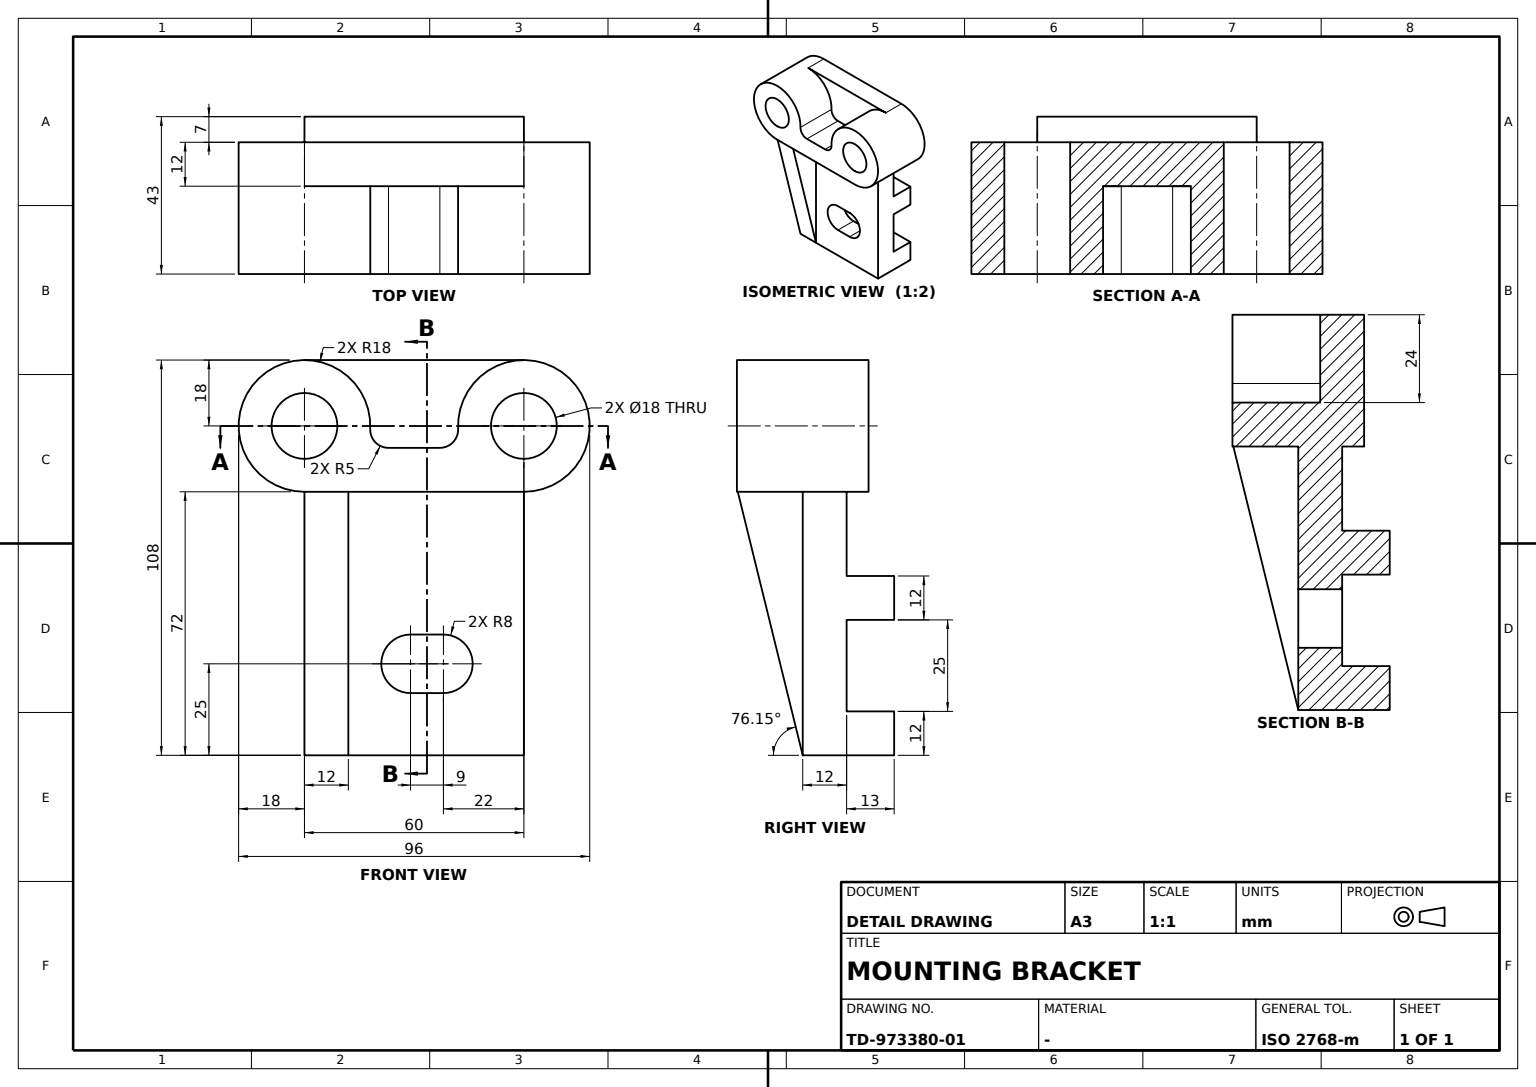
ISO-10303-21;
HEADER;
FILE_DESCRIPTION((''),'2;1');
FILE_NAME('','',(''),(''),'','','');
FILE_SCHEMA(('AUTOMOTIVE_DESIGN'));
ENDSEC;
DATA;
#1=APPLICATION_CONTEXT('');
#2=PRODUCT_CONTEXT('',#1,'mechanical');
#3=PRODUCT('','','',(#2));
#4=PRODUCT_DEFINITION_FORMATION('','',#3);
#5=PRODUCT_DEFINITION_CONTEXT('',#1,'design');
#6=PRODUCT_DEFINITION('','',#4,#5);
#7=PRODUCT_DEFINITION_SHAPE('','',#6);
#8=(LENGTH_UNIT()NAMED_UNIT(*)SI_UNIT(.MILLI.,.METRE.));
#9=(NAMED_UNIT(*)PLANE_ANGLE_UNIT()SI_UNIT($,.RADIAN.));
#10=(NAMED_UNIT(*)SI_UNIT($,.STERADIAN.)SOLID_ANGLE_UNIT());
#11=UNCERTAINTY_MEASURE_WITH_UNIT(LENGTH_MEASURE(0.005),#8,'distance_accuracy_value','');
#12=(GEOMETRIC_REPRESENTATION_CONTEXT(3)GLOBAL_UNCERTAINTY_ASSIGNED_CONTEXT((#11))GLOBAL_UNIT_ASSIGNED_CONTEXT((#8,#9,#10))REPRESENTATION_CONTEXT('',''));
#13=CARTESIAN_POINT('',(-18.,30.,45.));
#14=VERTEX_POINT('',#13);
#15=CARTESIAN_POINT('',(-18.,30.,54.));
#16=DIRECTION('',(1.,0.,0.));
#17=DIRECTION('',(0.,0.,-1.));
#18=AXIS2_PLACEMENT_3D('',#15,#16,#17);
#19=CIRCLE('',#18,9.);
#20=EDGE_CURVE('',#14,#14,#19,.T.);
#21=ORIENTED_EDGE('',*,*,#20,.F.);
#22=EDGE_LOOP('',(#21));
#23=FACE_BOUND('',#22,.T.);
#24=CARTESIAN_POINT('',(18.,30.,45.));
#25=VERTEX_POINT('',#24);
#26=CARTESIAN_POINT('',(18.,30.,54.));
#27=AXIS2_PLACEMENT_3D('',#26,#16,#17);
#28=CIRCLE('',#27,9.);
#29=EDGE_CURVE('',#25,#25,#28,.T.);
#30=ORIENTED_EDGE('',*,*,#29,.T.);
#31=EDGE_LOOP('',(#30));
#32=FACE_BOUND('',#31,.T.);
#33=CARTESIAN_POINT('',(0.,30.,54.));
#34=DIRECTION('',(0.,1.,0.));
#35=AXIS2_PLACEMENT_3D('',#33,#16,#34);
#36=CYLINDRICAL_SURFACE('',#35,9.);
#37=ADVANCED_FACE('',(#23,#32),#36,.F.);
#38=CARTESIAN_POINT('',(0.,-1.,-19.));
#39=VERTEX_POINT('',#38);
#40=CARTESIAN_POINT('',(0.,8.,-19.));
#41=VERTEX_POINT('',#40);
#42=CARTESIAN_POINT('',(0.,0.,-19.));
#43=VECTOR('',#34,1000.);
#44=LINE('',#42,#43);
#45=EDGE_CURVE('',#39,#41,#44,.T.);
#46=ORIENTED_EDGE('',*,*,#45,.T.);
#47=CARTESIAN_POINT('',(-12.,8.,-19.));
#48=VERTEX_POINT('',#47);
#49=CARTESIAN_POINT('',(-13.16,8.,-19.));
#50=VECTOR('',#16,1000.);
#51=LINE('',#49,#50);
#52=EDGE_CURVE('',#41,#48,#51,.F.);
#53=ORIENTED_EDGE('',*,*,#52,.T.);
#54=CARTESIAN_POINT('',(-12.,-1.,-19.));
#55=VERTEX_POINT('',#54);
#56=LINE('',#54,#43);
#57=EDGE_CURVE('',#55,#48,#56,.T.);
#58=ORIENTED_EDGE('',*,*,#57,.F.);
#59=CARTESIAN_POINT('',(-13.16,-1.,-19.));
#60=LINE('',#59,#50);
#61=EDGE_CURVE('',#39,#55,#60,.F.);
#62=ORIENTED_EDGE('',*,*,#61,.F.);
#63=EDGE_LOOP('',(#46,#53,#58,#62));
#64=FACE_BOUND('',#63,.T.);
#65=DIRECTION('',(0.,0.,1.));
#66=AXIS2_PLACEMENT_3D('',#38,#65,#34);
#67=PLANE('',#66);
#68=ADVANCED_FACE('',(#64),#67,.T.);
#69=CARTESIAN_POINT('',(-12.,-30.,13.));
#70=VERTEX_POINT('',#69);
#71=CARTESIAN_POINT('',(-25.,-30.,13.));
#72=VERTEX_POINT('',#71);
#73=CARTESIAN_POINT('',(0.,-30.,13.));
#74=DIRECTION('',(-1.,0.,0.));
#75=VECTOR('',#74,1000.);
#76=LINE('',#73,#75);
#77=EDGE_CURVE('',#70,#72,#76,.T.);
#78=ORIENTED_EDGE('',*,*,#77,.T.);
#79=CARTESIAN_POINT('',(-25.,-30.,1.));
#80=VERTEX_POINT('',#79);
#81=CARTESIAN_POINT('',(-25.,-30.,0.));
#82=VECTOR('',#17,1000.);
#83=LINE('',#81,#82);
#84=EDGE_CURVE('',#72,#80,#83,.T.);
#85=ORIENTED_EDGE('',*,*,#84,.T.);
#86=CARTESIAN_POINT('',(-12.,-30.,1.));
#87=VERTEX_POINT('',#86);
#88=CARTESIAN_POINT('',(0.,-30.,1.));
#89=LINE('',#88,#50);
#90=EDGE_CURVE('',#80,#87,#89,.T.);
#91=ORIENTED_EDGE('',*,*,#90,.T.);
#92=CARTESIAN_POINT('',(-12.,-30.,-24.));
#93=VERTEX_POINT('',#92);
#94=CARTESIAN_POINT('',(-12.,-30.,0.));
#95=LINE('',#94,#82);
#96=EDGE_CURVE('',#87,#93,#95,.T.);
#97=ORIENTED_EDGE('',*,*,#96,.T.);
#98=CARTESIAN_POINT('',(-25.,-30.,-24.));
#99=VERTEX_POINT('',#98);
#100=CARTESIAN_POINT('',(0.,-30.,-24.));
#101=LINE('',#100,#75);
#102=EDGE_CURVE('',#93,#99,#101,.T.);
#103=ORIENTED_EDGE('',*,*,#102,.T.);
#104=CARTESIAN_POINT('',(-25.,-30.,-36.));
#105=VERTEX_POINT('',#104);
#106=EDGE_CURVE('',#99,#105,#83,.T.);
#107=ORIENTED_EDGE('',*,*,#106,.T.);
#108=CARTESIAN_POINT('',(0.,-30.,-36.));
#109=VERTEX_POINT('',#108);
#110=LINE('',#108,#50);
#111=EDGE_CURVE('',#105,#109,#110,.T.);
#112=ORIENTED_EDGE('',*,*,#111,.T.);
#113=CARTESIAN_POINT('',(17.753425,-30.,36.));
#114=VERTEX_POINT('',#113);
#115=CARTESIAN_POINT('',(8.367946,-30.,-2.063329));
#116=DIRECTION('',(-0.239404888,0.,-0.970919822));
#117=VECTOR('',#116,1000.);
#118=LINE('',#115,#117);
#119=EDGE_CURVE('',#114,#109,#118,.T.);
#120=ORIENTED_EDGE('',*,*,#119,.F.);
#121=CARTESIAN_POINT('',(-12.,-30.,36.));
#122=VERTEX_POINT('',#121);
#123=CARTESIAN_POINT('',(0.,-30.,36.));
#124=LINE('',#123,#50);
#125=EDGE_CURVE('',#122,#114,#124,.T.);
#126=ORIENTED_EDGE('',*,*,#125,.F.);
#127=EDGE_CURVE('',#122,#70,#95,.T.);
#128=ORIENTED_EDGE('',*,*,#127,.T.);
#129=EDGE_LOOP('',(#78,#85,#91,#97,#103,#107,#112,#120,#126,#128));
#130=FACE_BOUND('',#129,.T.);
#131=CARTESIAN_POINT('',(0.,-30.,0.));
#132=AXIS2_PLACEMENT_3D('',#131,#34,#74);
#133=PLANE('',#132);
#134=ADVANCED_FACE('',(#130),#133,.F.);
#135=CARTESIAN_POINT('',(-18.,30.,36.));
#136=VERTEX_POINT('',#135);
#137=CARTESIAN_POINT('',(-12.,30.,36.));
#138=VERTEX_POINT('',#137);
#139=CARTESIAN_POINT('',(0.,30.,36.));
#140=LINE('',#139,#50);
#141=EDGE_CURVE('',#136,#138,#140,.T.);
#142=ORIENTED_EDGE('',*,*,#141,.T.);
#143=CARTESIAN_POINT('',(-12.,0.,36.));
#144=LINE('',#143,#43);
#145=EDGE_CURVE('',#122,#138,#144,.T.);
#146=ORIENTED_EDGE('',*,*,#145,.F.);
#147=CARTESIAN_POINT('',(-18.,-30.,36.));
#148=VERTEX_POINT('',#147);
#149=EDGE_CURVE('',#148,#122,#124,.T.);
#150=ORIENTED_EDGE('',*,*,#149,.F.);
#151=CARTESIAN_POINT('',(-18.,0.,36.));
#152=LINE('',#151,#43);
#153=EDGE_CURVE('',#148,#136,#152,.T.);
#154=ORIENTED_EDGE('',*,*,#153,.T.);
#155=EDGE_LOOP('',(#142,#146,#150,#154));
#156=FACE_BOUND('',#155,.T.);
#157=CARTESIAN_POINT('',(0.,0.,36.));
#158=AXIS2_PLACEMENT_3D('',#157,#17,#74);
#159=PLANE('',#158);
#160=ADVANCED_FACE('',(#156),#159,.T.);
#161=CARTESIAN_POINT('',(17.753425,-18.,36.));
#162=VERTEX_POINT('',#161);
#163=CARTESIAN_POINT('',(0.,-18.,-36.));
#164=VERTEX_POINT('',#163);
#165=CARTESIAN_POINT('',(18.,-18.,37.));
#166=LINE('',#165,#117);
#167=EDGE_CURVE('',#162,#164,#166,.T.);
#168=ORIENTED_EDGE('',*,*,#167,.T.);
#169=CARTESIAN_POINT('',(0.,-18.,36.));
#170=VERTEX_POINT('',#169);
#171=VECTOR('',#65,1000.);
#172=LINE('',#163,#171);
#173=EDGE_CURVE('',#164,#170,#172,.T.);
#174=ORIENTED_EDGE('',*,*,#173,.T.);
#175=LINE('',#169,#75);
#176=EDGE_CURVE('',#162,#170,#175,.T.);
#177=ORIENTED_EDGE('',*,*,#176,.F.);
#178=EDGE_LOOP('',(#168,#174,#177));
#179=FACE_BOUND('',#178,.T.);
#180=CARTESIAN_POINT('',(0.,-18.,0.));
#181=DIRECTION('',(0.,-1.,0.));
#182=AXIS2_PLACEMENT_3D('',#180,#181,#16);
#183=PLANE('',#182);
#184=ADVANCED_FACE('',(#179),#183,.F.);
#185=CARTESIAN_POINT('',(-12.,30.,1.));
#186=VERTEX_POINT('',#185);
#187=CARTESIAN_POINT('',(-12.,0.,1.));
#188=LINE('',#187,#43);
#189=EDGE_CURVE('',#87,#186,#188,.T.);
#190=ORIENTED_EDGE('',*,*,#189,.F.);
#191=ORIENTED_EDGE('',*,*,#90,.F.);
#192=CARTESIAN_POINT('',(-25.,30.,1.));
#193=VERTEX_POINT('',#192);
#194=CARTESIAN_POINT('',(-25.,0.,1.));
#195=LINE('',#194,#43);
#196=EDGE_CURVE('',#80,#193,#195,.T.);
#197=ORIENTED_EDGE('',*,*,#196,.T.);
#198=CARTESIAN_POINT('',(0.,30.,1.));
#199=LINE('',#198,#50);
#200=EDGE_CURVE('',#193,#186,#199,.T.);
#201=ORIENTED_EDGE('',*,*,#200,.T.);
#202=EDGE_LOOP('',(#190,#191,#197,#201));
#203=FACE_BOUND('',#202,.T.);
#204=AXIS2_PLACEMENT_3D('',#194,#65,#16);
#205=PLANE('',#204);
#206=ADVANCED_FACE('',(#203),#205,.F.);
#207=CARTESIAN_POINT('',(0.,0.,-36.));
#208=LINE('',#207,#43);
#209=EDGE_CURVE('',#109,#164,#208,.T.);
#210=ORIENTED_EDGE('',*,*,#209,.T.);
#211=ORIENTED_EDGE('',*,*,#167,.F.);
#212=LINE('',#113,#43);
#213=EDGE_CURVE('',#114,#162,#212,.T.);
#214=ORIENTED_EDGE('',*,*,#213,.F.);
#215=ORIENTED_EDGE('',*,*,#119,.T.);
#216=EDGE_LOOP('',(#210,#211,#214,#215));
#217=FACE_BOUND('',#216,.T.);
#218=CARTESIAN_POINT('',(18.,-30.,37.));
#219=DIRECTION('',(0.970919822,0.,-0.239404888));
#220=AXIS2_PLACEMENT_3D('',#218,#219,#116);
#221=PLANE('',#220);
#222=ADVANCED_FACE('',(#217),#221,.T.);
#223=CARTESIAN_POINT('',(0.,-1.,-3.));
#224=VERTEX_POINT('',#223);
#225=CARTESIAN_POINT('',(-12.,-1.,-3.));
#226=VERTEX_POINT('',#225);
#227=CARTESIAN_POINT('',(-13.16,-1.,-3.));
#228=LINE('',#227,#50);
#229=EDGE_CURVE('',#224,#226,#228,.F.);
#230=ORIENTED_EDGE('',*,*,#229,.F.);
#231=CARTESIAN_POINT('',(0.,-1.,-11.));
#232=AXIS2_PLACEMENT_3D('',#231,#74,#65);
#233=CIRCLE('',#232,8.);
#234=EDGE_CURVE('',#224,#39,#233,.F.);
#235=ORIENTED_EDGE('',*,*,#234,.T.);
#236=ORIENTED_EDGE('',*,*,#61,.T.);
#237=CARTESIAN_POINT('',(-12.,-1.,-11.));
#238=AXIS2_PLACEMENT_3D('',#237,#16,#17);
#239=CIRCLE('',#238,8.);
#240=EDGE_CURVE('',#226,#55,#239,.T.);
#241=ORIENTED_EDGE('',*,*,#240,.F.);
#242=EDGE_LOOP('',(#230,#235,#236,#241));
#243=FACE_BOUND('',#242,.T.);
#244=CARTESIAN_POINT('',(-13.16,-1.,-11.));
#245=AXIS2_PLACEMENT_3D('',#244,#16,#34);
#246=CYLINDRICAL_SURFACE('',#245,8.);
#247=ADVANCED_FACE('',(#243),#246,.F.);
#248=CARTESIAN_POINT('',(-6.,-7.021749,48.));
#249=VERTEX_POINT('',#248);
#250=CARTESIAN_POINT('',(-6.,-12.017021,53.217391));
#251=VERTEX_POINT('',#250);
#252=CARTESIAN_POINT('',(-6.,-7.021749,53.));
#253=AXIS2_PLACEMENT_3D('',#252,#74,#65);
#254=CIRCLE('',#253,5.);
#255=EDGE_CURVE('',#249,#251,#254,.T.);
#256=ORIENTED_EDGE('',*,*,#255,.T.);
#257=CARTESIAN_POINT('',(18.,-12.017021,53.217391));
#258=VERTEX_POINT('',#257);
#259=CARTESIAN_POINT('',(6.,-12.017021,53.217391));
#260=LINE('',#259,#75);
#261=EDGE_CURVE('',#258,#251,#260,.T.);
#262=ORIENTED_EDGE('',*,*,#261,.F.);
#263=CARTESIAN_POINT('',(18.,-7.021749,48.));
#264=VERTEX_POINT('',#263);
#265=CARTESIAN_POINT('',(18.,-7.021749,53.));
#266=AXIS2_PLACEMENT_3D('',#265,#16,#17);
#267=CIRCLE('',#266,5.);
#268=EDGE_CURVE('',#258,#264,#267,.T.);
#269=ORIENTED_EDGE('',*,*,#268,.T.);
#270=CARTESIAN_POINT('',(0.,-7.021749,48.));
#271=LINE('',#270,#75);
#272=EDGE_CURVE('',#264,#249,#271,.T.);
#273=ORIENTED_EDGE('',*,*,#272,.T.);
#274=EDGE_LOOP('',(#256,#262,#269,#273));
#275=FACE_BOUND('',#274,.T.);
#276=CARTESIAN_POINT('',(0.,-7.021749,53.));
#277=DIRECTION('',(0.,-0.999054373,0.043478261));
#278=AXIS2_PLACEMENT_3D('',#276,#74,#277);
#279=CYLINDRICAL_SURFACE('',#278,5.);
#280=ADVANCED_FACE('',(#275),#279,.F.);
#281=ORIENTED_EDGE('',*,*,#173,.F.);
#282=CARTESIAN_POINT('',(0.,30.,-36.));
#283=VERTEX_POINT('',#282);
#284=EDGE_CURVE('',#164,#283,#208,.T.);
#285=ORIENTED_EDGE('',*,*,#284,.T.);
#286=VERTEX_POINT('',#139);
#287=CARTESIAN_POINT('',(0.,30.,0.));
#288=LINE('',#287,#171);
#289=EDGE_CURVE('',#283,#286,#288,.T.);
#290=ORIENTED_EDGE('',*,*,#289,.T.);
#291=LINE('',#157,#43);
#292=EDGE_CURVE('',#170,#286,#291,.T.);
#293=ORIENTED_EDGE('',*,*,#292,.F.);
#294=EDGE_LOOP('',(#281,#285,#290,#293));
#295=FACE_BOUND('',#294,.T.);
#296=CARTESIAN_POINT('',(0.,8.,-3.));
#297=VERTEX_POINT('',#296);
#298=CARTESIAN_POINT('',(0.,0.,-3.));
#299=LINE('',#298,#43);
#300=EDGE_CURVE('',#224,#297,#299,.T.);
#301=ORIENTED_EDGE('',*,*,#300,.T.);
#302=CARTESIAN_POINT('',(0.,8.,-11.));
#303=AXIS2_PLACEMENT_3D('',#302,#74,#65);
#304=CIRCLE('',#303,8.);
#305=EDGE_CURVE('',#41,#297,#304,.F.);
#306=ORIENTED_EDGE('',*,*,#305,.F.);
#307=ORIENTED_EDGE('',*,*,#45,.F.);
#308=ORIENTED_EDGE('',*,*,#234,.F.);
#309=EDGE_LOOP('',(#301,#306,#307,#308));
#310=FACE_BOUND('',#309,.T.);
#311=AXIS2_PLACEMENT_3D('',#207,#74,#65);
#312=PLANE('',#311);
#313=ADVANCED_FACE('',(#295,#310),#312,.F.);
#314=CARTESIAN_POINT('',(-18.,-30.,45.));
#315=VERTEX_POINT('',#314);
#316=CARTESIAN_POINT('',(-18.,-30.,54.));
#317=AXIS2_PLACEMENT_3D('',#316,#16,#17);
#318=CIRCLE('',#317,9.);
#319=EDGE_CURVE('',#315,#315,#318,.T.);
#320=ORIENTED_EDGE('',*,*,#319,.F.);
#321=EDGE_LOOP('',(#320));
#322=FACE_BOUND('',#321,.T.);
#323=CARTESIAN_POINT('',(18.,-30.,45.));
#324=VERTEX_POINT('',#323);
#325=CARTESIAN_POINT('',(18.,-30.,54.));
#326=AXIS2_PLACEMENT_3D('',#325,#16,#17);
#327=CIRCLE('',#326,9.);
#328=EDGE_CURVE('',#324,#324,#327,.T.);
#329=ORIENTED_EDGE('',*,*,#328,.T.);
#330=EDGE_LOOP('',(#329));
#331=FACE_BOUND('',#330,.T.);
#332=CARTESIAN_POINT('',(0.,-30.,54.));
#333=AXIS2_PLACEMENT_3D('',#332,#16,#34);
#334=CYLINDRICAL_SURFACE('',#333,9.);
#335=ADVANCED_FACE('',(#322,#331),#334,.F.);
#336=ORIENTED_EDGE('',*,*,#111,.F.);
#337=CARTESIAN_POINT('',(-25.,30.,-36.));
#338=VERTEX_POINT('',#337);
#339=CARTESIAN_POINT('',(-25.,0.,-36.));
#340=LINE('',#339,#43);
#341=EDGE_CURVE('',#105,#338,#340,.T.);
#342=ORIENTED_EDGE('',*,*,#341,.T.);
#343=LINE('',#282,#50);
#344=EDGE_CURVE('',#338,#283,#343,.T.);
#345=ORIENTED_EDGE('',*,*,#344,.T.);
#346=ORIENTED_EDGE('',*,*,#284,.F.);
#347=ORIENTED_EDGE('',*,*,#209,.F.);
#348=EDGE_LOOP('',(#336,#342,#345,#346,#347));
#349=FACE_BOUND('',#348,.T.);
#350=AXIS2_PLACEMENT_3D('',#339,#65,#16);
#351=PLANE('',#350);
#352=ADVANCED_FACE('',(#349),#351,.F.);
#353=CARTESIAN_POINT('',(-18.,-30.,72.));
#354=VERTEX_POINT('',#353);
#355=CARTESIAN_POINT('',(-6.,-30.,72.));
#356=VERTEX_POINT('',#355);
#357=CARTESIAN_POINT('',(0.,-30.,72.));
#358=LINE('',#357,#50);
#359=EDGE_CURVE('',#354,#356,#358,.T.);
#360=ORIENTED_EDGE('',*,*,#359,.T.);
#361=CARTESIAN_POINT('',(-6.,30.,72.));
#362=VERTEX_POINT('',#361);
#363=VECTOR('',#181,1000.);
#364=LINE('',#361,#363);
#365=EDGE_CURVE('',#362,#356,#364,.T.);
#366=ORIENTED_EDGE('',*,*,#365,.F.);
#367=CARTESIAN_POINT('',(-18.,30.,72.));
#368=VERTEX_POINT('',#367);
#369=CARTESIAN_POINT('',(0.,30.,72.));
#370=LINE('',#369,#50);
#371=EDGE_CURVE('',#368,#362,#370,.T.);
#372=ORIENTED_EDGE('',*,*,#371,.F.);
#373=CARTESIAN_POINT('',(-18.,0.,72.));
#374=LINE('',#373,#363);
#375=EDGE_CURVE('',#368,#354,#374,.T.);
#376=ORIENTED_EDGE('',*,*,#375,.T.);
#377=EDGE_LOOP('',(#360,#366,#372,#376));
#378=FACE_BOUND('',#377,.T.);
#379=AXIS2_PLACEMENT_3D('',#367,#65,#181);
#380=PLANE('',#379);
#381=ADVANCED_FACE('',(#378),#380,.T.);
#382=ORIENTED_EDGE('',*,*,#125,.T.);
#383=CARTESIAN_POINT('',(18.,-30.,36.));
#384=VERTEX_POINT('',#383);
#385=EDGE_CURVE('',#114,#384,#124,.T.);
#386=ORIENTED_EDGE('',*,*,#385,.T.);
#387=CIRCLE('',#326,18.);
#388=EDGE_CURVE('',#258,#384,#387,.T.);
#389=ORIENTED_EDGE('',*,*,#388,.F.);
#390=ORIENTED_EDGE('',*,*,#261,.T.);
#391=CARTESIAN_POINT('',(-6.,-30.,54.));
#392=AXIS2_PLACEMENT_3D('',#391,#74,#65);
#393=CIRCLE('',#392,18.);
#394=EDGE_CURVE('',#356,#251,#393,.T.);
#395=ORIENTED_EDGE('',*,*,#394,.F.);
#396=ORIENTED_EDGE('',*,*,#359,.F.);
#397=CIRCLE('',#317,18.);
#398=EDGE_CURVE('',#354,#148,#397,.T.);
#399=ORIENTED_EDGE('',*,*,#398,.T.);
#400=ORIENTED_EDGE('',*,*,#149,.T.);
#401=EDGE_LOOP('',(#382,#386,#389,#390,#395,#396,#399,#400));
#402=FACE_BOUND('',#401,.T.);
#403=CYLINDRICAL_SURFACE('',#333,18.);
#404=ADVANCED_FACE('',(#402),#403,.T.);
#405=CARTESIAN_POINT('',(-12.,30.,-24.));
#406=VERTEX_POINT('',#405);
#407=CARTESIAN_POINT('',(-25.,30.,-24.));
#408=VERTEX_POINT('',#407);
#409=CARTESIAN_POINT('',(0.,30.,-24.));
#410=LINE('',#409,#75);
#411=EDGE_CURVE('',#406,#408,#410,.T.);
#412=ORIENTED_EDGE('',*,*,#411,.T.);
#413=CARTESIAN_POINT('',(-25.,0.,-24.));
#414=LINE('',#413,#43);
#415=EDGE_CURVE('',#99,#408,#414,.T.);
#416=ORIENTED_EDGE('',*,*,#415,.F.);
#417=ORIENTED_EDGE('',*,*,#102,.F.);
#418=CARTESIAN_POINT('',(-12.,0.,-24.));
#419=LINE('',#418,#43);
#420=EDGE_CURVE('',#93,#406,#419,.T.);
#421=ORIENTED_EDGE('',*,*,#420,.T.);
#422=EDGE_LOOP('',(#412,#416,#417,#421));
#423=FACE_BOUND('',#422,.T.);
#424=AXIS2_PLACEMENT_3D('',#418,#17,#74);
#425=PLANE('',#424);
#426=ADVANCED_FACE('',(#423),#425,.F.);
#427=ORIENTED_EDGE('',*,*,#29,.F.);
#428=EDGE_LOOP('',(#427));
#429=FACE_BOUND('',#428,.T.);
#430=ORIENTED_EDGE('',*,*,#328,.F.);
#431=EDGE_LOOP('',(#430));
#432=FACE_BOUND('',#431,.T.);
#433=ORIENTED_EDGE('',*,*,#388,.T.);
#434=CARTESIAN_POINT('',(18.,30.,36.));
#435=VERTEX_POINT('',#434);
#436=CARTESIAN_POINT('',(18.,0.,36.));
#437=LINE('',#436,#43);
#438=EDGE_CURVE('',#384,#435,#437,.T.);
#439=ORIENTED_EDGE('',*,*,#438,.T.);
#440=CARTESIAN_POINT('',(18.,12.017021,53.217391));
#441=VERTEX_POINT('',#440);
#442=CIRCLE('',#27,18.);
#443=EDGE_CURVE('',#435,#441,#442,.T.);
#444=ORIENTED_EDGE('',*,*,#443,.T.);
#445=CARTESIAN_POINT('',(18.,7.021749,48.));
#446=VERTEX_POINT('',#445);
#447=CARTESIAN_POINT('',(18.,7.021749,53.));
#448=AXIS2_PLACEMENT_3D('',#447,#16,#17);
#449=CIRCLE('',#448,5.);
#450=EDGE_CURVE('',#446,#441,#449,.T.);
#451=ORIENTED_EDGE('',*,*,#450,.F.);
#452=CARTESIAN_POINT('',(18.,0.,48.));
#453=LINE('',#452,#43);
#454=EDGE_CURVE('',#264,#446,#453,.T.);
#455=ORIENTED_EDGE('',*,*,#454,.F.);
#456=ORIENTED_EDGE('',*,*,#268,.F.);
#457=EDGE_LOOP('',(#433,#439,#444,#451,#455,#456));
#458=FACE_BOUND('',#457,.T.);
#459=CARTESIAN_POINT('',(18.,0.,0.));
#460=AXIS2_PLACEMENT_3D('',#459,#16,#34);
#461=PLANE('',#460);
#462=ADVANCED_FACE('',(#429,#432,#458),#461,.T.);
#463=EDGE_CURVE('',#286,#435,#140,.T.);
#464=ORIENTED_EDGE('',*,*,#463,.T.);
#465=ORIENTED_EDGE('',*,*,#438,.F.);
#466=ORIENTED_EDGE('',*,*,#385,.F.);
#467=ORIENTED_EDGE('',*,*,#213,.T.);
#468=ORIENTED_EDGE('',*,*,#176,.T.);
#469=ORIENTED_EDGE('',*,*,#292,.T.);
#470=EDGE_LOOP('',(#464,#465,#466,#467,#468,#469));
#471=FACE_BOUND('',#470,.T.);
#472=ADVANCED_FACE('',(#471),#159,.T.);
#473=ORIENTED_EDGE('',*,*,#52,.F.);
#474=ORIENTED_EDGE('',*,*,#305,.T.);
#475=CARTESIAN_POINT('',(-12.,8.,-3.));
#476=VERTEX_POINT('',#475);
#477=CARTESIAN_POINT('',(-13.16,8.,-3.));
#478=LINE('',#477,#50);
#479=EDGE_CURVE('',#297,#476,#478,.F.);
#480=ORIENTED_EDGE('',*,*,#479,.T.);
#481=CARTESIAN_POINT('',(-12.,8.,-11.));
#482=AXIS2_PLACEMENT_3D('',#481,#16,#17);
#483=CIRCLE('',#482,8.);
#484=EDGE_CURVE('',#48,#476,#483,.T.);
#485=ORIENTED_EDGE('',*,*,#484,.F.);
#486=EDGE_LOOP('',(#473,#474,#480,#485));
#487=FACE_BOUND('',#486,.T.);
#488=CARTESIAN_POINT('',(-13.16,8.,-11.));
#489=AXIS2_PLACEMENT_3D('',#488,#16,#34);
#490=CYLINDRICAL_SURFACE('',#489,8.);
#491=ADVANCED_FACE('',(#487),#490,.F.);
#492=ORIENTED_EDGE('',*,*,#272,.F.);
#493=ORIENTED_EDGE('',*,*,#454,.T.);
#494=CARTESIAN_POINT('',(-6.,7.021749,48.));
#495=VERTEX_POINT('',#494);
#496=CARTESIAN_POINT('',(0.,7.021749,48.));
#497=LINE('',#496,#75);
#498=EDGE_CURVE('',#446,#495,#497,.T.);
#499=ORIENTED_EDGE('',*,*,#498,.T.);
#500=CARTESIAN_POINT('',(-6.,0.,48.));
#501=LINE('',#500,#363);
#502=EDGE_CURVE('',#495,#249,#501,.T.);
#503=ORIENTED_EDGE('',*,*,#502,.T.);
#504=EDGE_LOOP('',(#492,#493,#499,#503));
#505=FACE_BOUND('',#504,.T.);
#506=CARTESIAN_POINT('',(0.,-13.029438,48.));
#507=AXIS2_PLACEMENT_3D('',#506,#17,#34);
#508=PLANE('',#507);
#509=ADVANCED_FACE('',(#505),#508,.F.);
#510=ORIENTED_EDGE('',*,*,#145,.T.);
#511=CARTESIAN_POINT('',(-12.,30.,13.));
#512=VERTEX_POINT('',#511);
#513=CARTESIAN_POINT('',(-12.,30.,0.));
#514=LINE('',#513,#82);
#515=EDGE_CURVE('',#138,#512,#514,.T.);
#516=ORIENTED_EDGE('',*,*,#515,.T.);
#517=CARTESIAN_POINT('',(-12.,0.,13.));
#518=LINE('',#517,#43);
#519=EDGE_CURVE('',#70,#512,#518,.T.);
#520=ORIENTED_EDGE('',*,*,#519,.F.);
#521=ORIENTED_EDGE('',*,*,#127,.F.);
#522=EDGE_LOOP('',(#510,#516,#520,#521));
#523=FACE_BOUND('',#522,.T.);
#524=AXIS2_PLACEMENT_3D('',#187,#16,#17);
#525=PLANE('',#524);
#526=ADVANCED_FACE('',(#523),#525,.F.);
#527=ORIENTED_EDGE('',*,*,#196,.F.);
#528=ORIENTED_EDGE('',*,*,#84,.F.);
#529=CARTESIAN_POINT('',(-25.,30.,13.));
#530=VERTEX_POINT('',#529);
#531=CARTESIAN_POINT('',(-25.,0.,13.));
#532=LINE('',#531,#43);
#533=EDGE_CURVE('',#72,#530,#532,.T.);
#534=ORIENTED_EDGE('',*,*,#533,.T.);
#535=CARTESIAN_POINT('',(-25.,30.,0.));
#536=LINE('',#535,#82);
#537=EDGE_CURVE('',#530,#193,#536,.T.);
#538=ORIENTED_EDGE('',*,*,#537,.T.);
#539=EDGE_LOOP('',(#527,#528,#534,#538));
#540=FACE_BOUND('',#539,.T.);
#541=AXIS2_PLACEMENT_3D('',#413,#16,#17);
#542=PLANE('',#541);
#543=ADVANCED_FACE('',(#540),#542,.F.);
#544=LINE('',#225,#43);
#545=EDGE_CURVE('',#226,#476,#544,.T.);
#546=ORIENTED_EDGE('',*,*,#545,.T.);
#547=ORIENTED_EDGE('',*,*,#479,.F.);
#548=ORIENTED_EDGE('',*,*,#300,.F.);
#549=ORIENTED_EDGE('',*,*,#229,.T.);
#550=EDGE_LOOP('',(#546,#547,#548,#549));
#551=FACE_BOUND('',#550,.T.);
#552=AXIS2_PLACEMENT_3D('',#223,#65,#34);
#553=PLANE('',#552);
#554=ADVANCED_FACE('',(#551),#553,.F.);
#555=ORIENTED_EDGE('',*,*,#371,.T.);
#556=CARTESIAN_POINT('',(-6.,12.017021,53.217391));
#557=VERTEX_POINT('',#556);
#558=CARTESIAN_POINT('',(-6.,30.,54.));
#559=AXIS2_PLACEMENT_3D('',#558,#74,#65);
#560=CIRCLE('',#559,18.);
#561=EDGE_CURVE('',#557,#362,#560,.T.);
#562=ORIENTED_EDGE('',*,*,#561,.F.);
#563=CARTESIAN_POINT('',(6.,12.017021,53.217391));
#564=LINE('',#563,#50);
#565=EDGE_CURVE('',#441,#557,#564,.F.);
#566=ORIENTED_EDGE('',*,*,#565,.F.);
#567=ORIENTED_EDGE('',*,*,#443,.F.);
#568=ORIENTED_EDGE('',*,*,#463,.F.);
#569=LINE('',#137,#50);
#570=EDGE_CURVE('',#138,#286,#569,.T.);
#571=ORIENTED_EDGE('',*,*,#570,.F.);
#572=ORIENTED_EDGE('',*,*,#141,.F.);
#573=CIRCLE('',#18,18.);
#574=EDGE_CURVE('',#136,#368,#573,.T.);
#575=ORIENTED_EDGE('',*,*,#574,.T.);
#576=EDGE_LOOP('',(#555,#562,#566,#567,#568,#571,#572,#575));
#577=FACE_BOUND('',#576,.T.);
#578=CYLINDRICAL_SURFACE('',#35,18.);
#579=ADVANCED_FACE('',(#577),#578,.T.);
#580=CARTESIAN_POINT('',(0.,30.,13.));
#581=LINE('',#580,#75);
#582=EDGE_CURVE('',#512,#530,#581,.T.);
#583=ORIENTED_EDGE('',*,*,#582,.F.);
#584=ORIENTED_EDGE('',*,*,#515,.F.);
#585=ORIENTED_EDGE('',*,*,#570,.T.);
#586=ORIENTED_EDGE('',*,*,#289,.F.);
#587=ORIENTED_EDGE('',*,*,#344,.F.);
#588=EDGE_CURVE('',#408,#338,#536,.T.);
#589=ORIENTED_EDGE('',*,*,#588,.F.);
#590=ORIENTED_EDGE('',*,*,#411,.F.);
#591=EDGE_CURVE('',#186,#406,#514,.T.);
#592=ORIENTED_EDGE('',*,*,#591,.F.);
#593=ORIENTED_EDGE('',*,*,#200,.F.);
#594=ORIENTED_EDGE('',*,*,#537,.F.);
#595=EDGE_LOOP('',(#583,#584,#585,#586,#587,#589,#590,#592,#593,#594));
#596=FACE_BOUND('',#595,.T.);
#597=AXIS2_PLACEMENT_3D('',#287,#34,#74);
#598=PLANE('',#597);
#599=ADVANCED_FACE('',(#596),#598,.T.);
#600=ORIENTED_EDGE('',*,*,#450,.T.);
#601=ORIENTED_EDGE('',*,*,#565,.T.);
#602=CARTESIAN_POINT('',(-6.,7.021749,53.));
#603=AXIS2_PLACEMENT_3D('',#602,#74,#65);
#604=CIRCLE('',#603,5.);
#605=EDGE_CURVE('',#557,#495,#604,.T.);
#606=ORIENTED_EDGE('',*,*,#605,.T.);
#607=ORIENTED_EDGE('',*,*,#498,.F.);
#608=EDGE_LOOP('',(#600,#601,#606,#607));
#609=FACE_BOUND('',#608,.T.);
#610=CARTESIAN_POINT('',(0.,7.021749,53.));
#611=AXIS2_PLACEMENT_3D('',#610,#74,#17);
#612=CYLINDRICAL_SURFACE('',#611,5.);
#613=ADVANCED_FACE('',(#609),#612,.F.);
#614=ORIENTED_EDGE('',*,*,#77,.F.);
#615=ORIENTED_EDGE('',*,*,#519,.T.);
#616=ORIENTED_EDGE('',*,*,#582,.T.);
#617=ORIENTED_EDGE('',*,*,#533,.F.);
#618=EDGE_LOOP('',(#614,#615,#616,#617));
#619=FACE_BOUND('',#618,.T.);
#620=AXIS2_PLACEMENT_3D('',#517,#17,#74);
#621=PLANE('',#620);
#622=ADVANCED_FACE('',(#619),#621,.F.);
#623=ORIENTED_EDGE('',*,*,#319,.T.);
#624=EDGE_LOOP('',(#623));
#625=FACE_BOUND('',#624,.T.);
#626=ORIENTED_EDGE('',*,*,#398,.F.);
#627=ORIENTED_EDGE('',*,*,#375,.F.);
#628=ORIENTED_EDGE('',*,*,#574,.F.);
#629=ORIENTED_EDGE('',*,*,#153,.F.);
#630=EDGE_LOOP('',(#626,#627,#628,#629));
#631=FACE_BOUND('',#630,.T.);
#632=ORIENTED_EDGE('',*,*,#20,.T.);
#633=EDGE_LOOP('',(#632));
#634=FACE_BOUND('',#633,.T.);
#635=CARTESIAN_POINT('',(-18.,0.,0.));
#636=AXIS2_PLACEMENT_3D('',#635,#16,#34);
#637=PLANE('',#636);
#638=ADVANCED_FACE('',(#625,#631,#634),#637,.F.);
#639=ORIENTED_EDGE('',*,*,#96,.F.);
#640=ORIENTED_EDGE('',*,*,#189,.T.);
#641=ORIENTED_EDGE('',*,*,#591,.T.);
#642=ORIENTED_EDGE('',*,*,#420,.F.);
#643=EDGE_LOOP('',(#639,#640,#641,#642));
#644=FACE_BOUND('',#643,.T.);
#645=ORIENTED_EDGE('',*,*,#484,.T.);
#646=ORIENTED_EDGE('',*,*,#545,.F.);
#647=ORIENTED_EDGE('',*,*,#240,.T.);
#648=ORIENTED_EDGE('',*,*,#57,.T.);
#649=EDGE_LOOP('',(#645,#646,#647,#648));
#650=FACE_BOUND('',#649,.T.);
#651=ADVANCED_FACE('',(#644,#650),#525,.F.);
#652=ORIENTED_EDGE('',*,*,#605,.F.);
#653=ORIENTED_EDGE('',*,*,#561,.T.);
#654=ORIENTED_EDGE('',*,*,#365,.T.);
#655=ORIENTED_EDGE('',*,*,#394,.T.);
#656=ORIENTED_EDGE('',*,*,#255,.F.);
#657=ORIENTED_EDGE('',*,*,#502,.F.);
#658=EDGE_LOOP('',(#652,#653,#654,#655,#656,#657));
#659=FACE_BOUND('',#658,.T.);
#660=CARTESIAN_POINT('',(-6.,0.,0.));
#661=AXIS2_PLACEMENT_3D('',#660,#74,#181);
#662=PLANE('',#661);
#663=ADVANCED_FACE('',(#659),#662,.F.);
#664=ORIENTED_EDGE('',*,*,#106,.F.);
#665=ORIENTED_EDGE('',*,*,#415,.T.);
#666=ORIENTED_EDGE('',*,*,#588,.T.);
#667=ORIENTED_EDGE('',*,*,#341,.F.);
#668=EDGE_LOOP('',(#664,#665,#666,#667));
#669=FACE_BOUND('',#668,.T.);
#670=ADVANCED_FACE('',(#669),#542,.F.);
#671=CLOSED_SHELL('',(#37,#68,#134,#160,#184,#206,#222,#247,#280,#313,#335,#352,#381,#404,#426,#462,#472,#491,#509,#526,#543,#554,#579,#599,#613,#622,#638,#651,#663,#670));
#672=MANIFOLD_SOLID_BREP('',#671);
#673=ADVANCED_BREP_SHAPE_REPRESENTATION('',(#672),#12);
#674=SHAPE_DEFINITION_REPRESENTATION(#7,#673);
ENDSEC;
END-ISO-10303-21;
